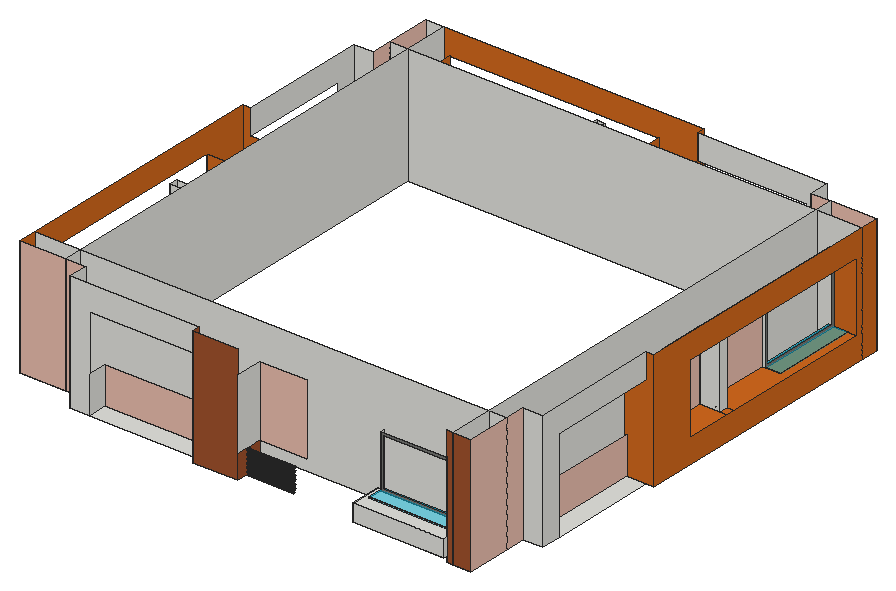
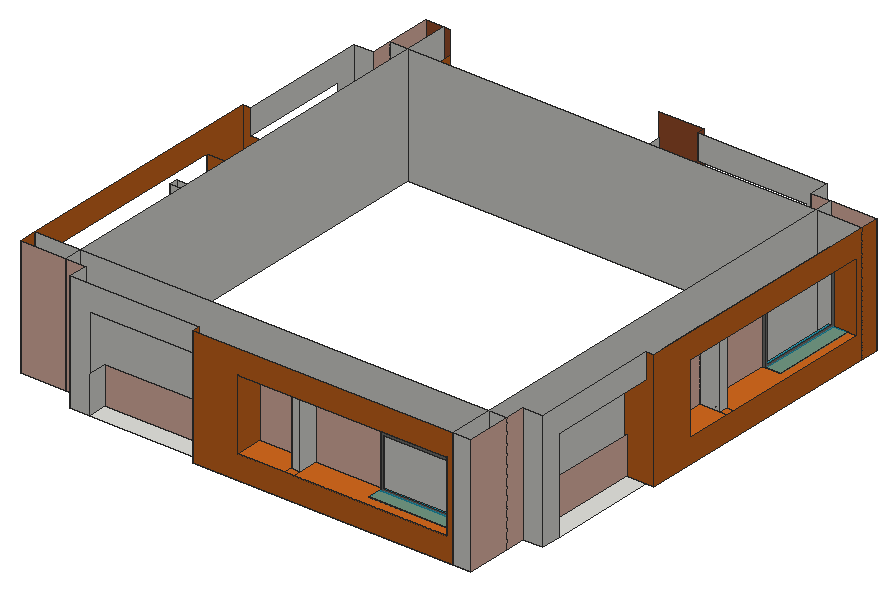
# SketchUp Ruby script. Lengths in inches.
U = 1.inch
M = Sketchup.active_model
def pt(a) = Geom::Point3d.new(a.map { |v| v * U })
def face(e, loops, mat)
  f = e.add_face(loops[0].map { |a| pt(a) })
  loops[1..].each { |l| e.add_face(l.map { |a| pt(a) }).erase! }
  f.material = f.back_material = mat if mat
  f
end
# faces: each face lists its corners as indices into pts; further lists are holes
def faces(e, pts, list, mat = nil) = list.each { |f| face(e, (f[0].is_a?(Array) ? f : [f]).map { |l| l.map { |i| pts[i] } }, mat) }
# xy, xz, yz: faces in a plane at the given z, y or x. An outline is a flat list of corners, or four numbers for a rectangle; further outlines are holes
def ring(l) = l.size == 4 ? [[l[0], l[1]], [l[2], l[1]], [l[2], l[3]], [l[0], l[3]]] : l.each_slice(2).to_a
def flat(e, list, mat, &to3) = list.each { |f| face(e, (f[0].is_a?(Array) ? f : [f]).map { |l| ring(l).map { |u, v| to3.(u, v) } }, mat) }
def xy(e, z, list, mat = nil) = flat(e, list, mat) { |x, y| [x, y, z] }
def xz(e, y, list, mat = nil) = flat(e, list, mat) { |x, z| [x, y, z] }
def yz(e, x, list, mat = nil) = flat(e, list, mat) { |y, z| [x, y, z] }
def lines(e, pts, list) = list.each { |a, b| e.add_line(pt(pts[a]), pt(pts[b])) }
# prism: a flat outline (further loops are holes) pulled along v
def prism(e, loops, v, mat = nil)
  f = face(e, loops, mat); d = Geom::Vector3d.new(v.map { |x| x * U })
  f.pushpull(f.normal.samedirection?(d) ? d.length : -d.length)
end
def box(e, o, s, mat = nil) = prism(e, [[o, [o[0] + s[0], o[1], o[2]], [o[0] + s[0], o[1] + s[1], o[2]], [o[0], o[1] + s[1], o[2]]]], [0, 0, s[2]], mat)
def at(x, y, z, deg = 0) = Geom::Transformation.translation(pt([x, y, z])) * Geom::Transformation.rotation(ORIGIN, Z_AXIS, deg.degrees)
def axes(o, x, y, z) = Geom::Transformation.new([*x, 0, *y, 0, *z, 0, *pt(o).to_a, 1])
def part(name) = M.definitions.add(name)
# library, detail: a bought-in or finely detailed component or shape, given as its bounding box
def library(name, o, s) = part(name).tap { |d| box(d.entities, o, s) }
def detail(e, o, s) = box(e.add_group.entities, o, s)
def put(e, d, t, mat = nil) = e.add_instance(d, t).tap { |i| i.material = mat if mat }
def group(e, t, mat = nil) = e.add_group.tap { |g| g.transformation = t; g.material = mat if mat }.entities
root = M.entities
M.materials.add("[0041_Chocolate]").color = [210, 105, 30]
M.materials.add("[0042_Sienna]").color = [160, 82, 45]
M.materials.add("[0119_RosyBrown]").color = [234, 190, 174]
M.materials.add("[Metal Seamed]").color = [118, 119, 115]
M.materials.add("[Translucent Glass Tinted]").color = [8, 201, 241]
M.materials["[Translucent Glass Tinted]"].alpha = 0.48
c1 = part("Altan")
box(c1.entities,[0,0,0],[118.11,59.06,3.9375])
prism(root,[[[1139,96.8125,797.98],[1414.89,97.68,797.98],[1415.2,0.87,797.98],[1139.3,0,797.98]]],[0,0,52.19])
xy(root,780,[[1434.3125,12.8125,1488,150.5],[306.65,36.8125,641.22,96.8125],[48,96.8125,185.6875,150.5],[48,150.5,185.6875,150.5,185.6875,1399.125,132,1399.125,132,1338.16,72,1338.16,72,1278.16,132,1278.16,132,943.59,48,943.59],[1434.3125,150.5,1488,150.5,1488,211.46,1548,211.46,1548,271.47,1488,271.47,1488,606.03,1572,606.03,1572,1399.125,1434.3125,1399.125],
  [1488,271.47,1548,606.03],[72,943.59,132,1278.16],[132,1399.125,185.6875,1536.8125],[185.6875,1399.125,1434.3125,1399.125,1434.3125,1452.8125,1373.35,1452.8125,1373.35,1512.8125,1313.35,1512.8125,1313.35,1452.8125,978.78,1452.8125,978.78,1536.8125,185.6875,1536.8125],[1434.3125,1399.125,1572,1452.8125],
  [978.78,1452.8125,1313.35,1512.8125]])
xy(root,853.11,[[72,636.29,132,662.8],[1488,886.83,1548,913.33],[671.48,1452.8125,697.99,1512.8125]])
xy(root,853.11,[[48,169.92,120,169.92,120,429.61,132,429.61,132,636.29,48,636.29],[48,636.29,72,662.8],[48,662.8,132,806.17],[1488,743.45,1572,886.83],[1548,886.83,1572,913.33],
  [1488,913.33,1572,913.33,1572,1379.7,1500,1379.7,1500,1120.01,1488,1120.01],[464.8,1452.8125,671.48,1452.8125,671.48,1536.8125,205.11,1536.8125,205.11,1464.8125,464.8,1464.8125],[697.99,1452.8125,841.36,1536.8125],[671.48,1512.8125,697.99,1536.8125]],"[0041_Chocolate]")
xy(root,853.11,[[1155.2,84.8125,1414.89,96.8125]],"[0042_Sienna]")
xz(root,12.8125,[[641.22,780,778.64,1140],[1414.89,780,1434.3125,1140],[1434.3125,780,1488,1140]],"[0042_Sienna]")
xz(root,36.8125,[[246.65,780,306.65,780,306.65,1062.625,641.22,1062.625,641.22,1140,246.65,1140]])
xz(root,84.8125,[[[1155.2,853.11,1414.89,1013.61],[1161.2,859.11,1408.89,1007.61]]],"[Metal Seamed]")
xz(root,96.8125,[[48,780,185.6875,1140],[185.6875,780,246.65,1140],[306.65,780,641.22,893.76],[778.64,853.11,922.01,1066.89]],"[0119_RosyBrown]")
xz(root,150.5,[[48,780,1488,1140]])
xz(root,169.92,[[48,853.11,48,1066.89,132,1066.89,132,1013.61,120,1013.61,120,853.11]],"[0041_Chocolate]")
xz(root,211.46,[[1488,780,1548,1140]])
xz(root,271.47,[[1488,780,1548,893.76]])
xz(root,429.61,[[120,853.11,132,1013.61]],"[Metal Seamed]")
xz(root,606.03,[[1488,780,1572,780,1572,1140,1548,1140,1548,1062.625,1482,1062.625,1482,893.76,1488,893.76]],"[0041_Chocolate]")
xz(root,636.29,[[72,853.11,132,1066.89]])
xz(root,662.8,[[[72,853.11,132,1066.89],[83.53,858.02,84.48,858.14,85.37,858.51,86.13,859.1,86.72,859.86,87.09,860.75,87.21,861.7,87.09,862.66,86.72,863.55,86.13,864.3125,85.37,864.9,84.48,865.27,83.53,865.39,82.57,865.27,81.68,864.9,80.92,864.3125,80.33,863.55,79.97,862.66,79.84,861.7,79.97,860.75,80.33,859.86,80.92,859.1,81.68,858.51,82.57,858.14]]])
xz(root,743.45,[[[1488,853.11,1572,1066.89],[1536.47,858.02,1537.43,858.14,1538.32,858.51,1539.08,859.1,1539.67,859.86,1540.03,860.75,1540.16,861.7,1540.03,862.66,1539.67,863.55,1539.08,864.3125,1538.32,864.9,1537.43,865.27,1536.47,865.39,1535.52,865.27,1534.63,864.9,1533.87,864.3125,1533.28,863.55,1532.91,862.66,1532.79,861.7,1532.91,860.75,1533.28,859.86,1533.87,859.1,1534.63,858.51,1535.52,858.14]]],"[0041_Chocolate]")
xz(root,806.17,[[[48,853.11,132,1066.89],[83.53,858.02,82.57,858.14,81.68,858.51,80.92,859.1,80.33,859.86,79.97,860.75,79.84,861.7,79.97,862.66,80.33,863.55,80.92,864.3125,81.68,864.9,82.57,865.27,83.53,865.39,84.48,865.27,85.37,864.9,86.13,864.3125,86.72,863.55,87.09,862.66,87.21,861.7,87.09,860.75,86.72,859.86,86.13,859.1,85.37,858.51,84.48,858.14]]],"[0041_Chocolate]")
xz(root,886.83,[[[1488,853.11,1548,1066.89],[1536.47,858.02,1535.52,858.14,1534.63,858.51,1533.87,859.1,1533.28,859.86,1532.91,860.75,1532.79,861.7,1532.91,862.66,1533.28,863.55,1533.87,864.3125,1534.63,864.9,1535.52,865.27,1536.47,865.39,1537.43,865.27,1538.32,864.9,1539.08,864.3125,1539.67,863.55,1540.03,862.66,1540.16,861.7,1540.03,860.75,1539.67,859.86,1539.08,859.1,1538.32,858.51,1537.43,858.14]]])
xz(root,913.33,[[1488,853.11,1548,1066.89]])
xz(root,943.59,[[48,780,48,1140,72,1140,72,1062.625,138,1062.625,138,893.76,132,893.76,132,780]],"[0041_Chocolate]")
xz(root,1120.01,[[1488,853.11,1500,1013.61]])
xz(root,1278.16,[[72,780,132,893.76]])
xz(root,1338.16,[[72,780,132,1140]])
xz(root,1379.7,[[1500,853.11,1572,853.11,1572,1066.89,1488,1066.89,1488,1013.61,1500,1013.61]],"[0041_Chocolate]")
xz(root,1399.125,[[132,780,1572,1140]])
xz(root,1452.8125,[[671.48,853.11,697.99,1066.89]])
xz(root,1452.8125,[[978.78,780,1313.35,893.76],[1373.35,780,1434.3125,1140],[1434.3125,780,1572,1140],[464.8,853.11,464.8,1013.61,205.11,1013.61,205.11,1066.89,671.48,1066.89,671.48,853.11],[697.99,853.11,841.36,1066.89]],"[0119_RosyBrown]")
xz(root,1464.8125,[[[205.11,853.11,464.8,1013.61],[211.11,859.11,458.8,1007.61]]],"[Metal Seamed]")
xz(root,1512.8125,[[1313.35,780,1313.35,1062.625,978.78,1062.625,978.78,1140,1373.35,1140,1373.35,780],[671.48,853.11,697.99,1066.89]])
xz(root,1536.8125,[[132,780,185.6875,1140]])
xz(root,1536.8125,[[[185.6875,780,978.78,1140],[205.11,853.11,841.36,1066.89]]],"[0041_Chocolate]")
yz(root,48,[[96.8125,780,150.5,1140],[[150.5,780,943.59,1140],[169.92,853.11,806.17,1066.89]]],"[0041_Chocolate]")
yz(root,72,[[1278.16,780,1278.16,1062.625,943.59,1062.625,943.59,1140,1338.16,1140,1338.16,780],[636.29,853.11,662.8,1066.89]])
yz(root,120,[[[169.92,853.11,429.61,1013.61],[175.92,859.11,423.61,1007.61]]],"[Metal Seamed]")
yz(root,132,[[636.29,853.11,662.8,1066.89]])
yz(root,132,[[943.59,780,1278.16,893.76],[1338.16,780,1399.125,1140],[1399.125,780,1536.8125,1140],[429.61,853.11,429.61,1013.61,169.92,1013.61,169.92,1066.89,636.29,1066.89,636.29,853.11],[662.8,853.11,806.17,1066.89]],"[0119_RosyBrown]")
yz(root,185.6875,[[96.8125,780,1536.8125,1140]])
yz(root,205.11,[[1464.8125,853.11,1536.8125,853.11,1536.8125,1066.89,1452.8125,1066.89,1452.8125,1013.61,1464.8125,1013.61]],"[0041_Chocolate]")
yz(root,246.65,[[36.8125,780,96.8125,1140]])
yz(root,306.65,[[36.8125,780,96.8125,893.76]])
yz(root,464.8,[[1452.8125,853.11,1464.8125,1013.61]])
yz(root,641.22,[[12.8125,780,12.8125,1140,36.8125,1140,36.8125,1062.625,102.8125,1062.625,102.8125,893.76,96.8125,893.76,96.8125,780]],"[0042_Sienna]")
yz(root,671.48,[[1452.8125,853.11,1512.8125,1066.89]])
yz(root,697.99,[[[1452.8125,853.11,1512.8125,1066.89],[1501.28,858.02,1500.33,858.14,1499.44,858.51,1498.68,859.1,1498.09,859.86,1497.72,860.75,1497.6,861.7,1497.72,862.66,1498.09,863.55,1498.68,864.3125,1499.44,864.9,1500.33,865.27,1501.28,865.39,1502.24,865.27,1503.13,864.9,1503.89,864.3125,1504.48,863.55,1504.85,862.66,1504.97,861.7,1504.85,860.75,1504.48,859.86,1503.89,859.1,1503.13,858.51,1502.24,858.14]]])
yz(root,778.64,[[[12.8125,853.11,47.01,853.11,47.38,853.27,48.34,853.39,49.29,853.27,49.67,853.11,96.8125,853.11,96.8125,1066.89,51.8,1066.89,51.9,1066.66,52.03,1065.7,51.9,1064.75,51.53,1063.86,50.95,1063.1,50.18,1062.51,49.29,1062.14,48.34,1062.02,47.38,1062.14,46.5,1062.51,45.73,1063.1,45.15,1063.86,44.78,1064.75,44.65,1065.7,44.78,1066.66,44.875,1066.89,12.8125,1066.89],[48.34,858.02,47.38,858.14,46.5,858.51,45.73,859.1,45.15,859.86,44.78,860.75,44.65,861.7,44.78,862.66,45.15,863.55,45.73,864.3125,46.5,864.9,47.38,865.27,48.34,865.39,49.29,865.27,50.18,864.9,50.95,864.3125,51.53,863.55,51.9,862.66,52.03,861.7,51.9,860.75,51.53,859.86,50.95,859.1,50.18,858.51,49.29,858.14]],[47.01,853.11,49.67,853.11,49.29,853.27,48.34,853.39,47.38,853.27]])
yz(root,778.64,[[12.8125,780,45.49,780,45.73,780.3125,46.5,780.9,47.38,781.27,48.34,781.39,49.29,781.27,50.18,780.9,50.95,780.3125,51.19,780,96.8125,780,96.8125,853.11,49.67,853.11,50.18,852.9,50.95,852.3125,51.53,851.55,51.9,850.66,52.03,849.7,51.9,848.75,51.53,847.86,50.95,847.1,50.18,846.51,49.29,846.14,48.34,846.02,47.38,846.14,46.5,846.51,45.73,847.1,45.15,847.86,44.78,848.75,44.65,849.7,44.78,850.66,45.15,851.55,45.73,852.3125,46.5,852.9,47.01,853.11,12.8125,853.11],[45.49,780,51.19,780,50.95,780.3125,50.18,780.9,49.29,781.27,48.34,781.39,47.38,781.27,46.5,780.9,45.73,780.3125],[48.34,846.02,49.29,846.14,50.18,846.51,50.95,847.1,51.53,847.86,51.9,848.75,52.03,849.7,51.9,850.66,51.53,851.55,50.95,852.3125,50.18,852.9,49.67,853.11,47.01,853.11,46.5,852.9,45.73,852.3125,45.15,851.55,44.78,850.66,44.65,849.7,44.78,848.75,45.15,847.86,45.73,847.1,46.5,846.51,47.38,846.14]],"[0042_Sienna]")
yz(root,841.36,[[[1452.8125,853.11,1536.8125,1066.89],[1501.28,858.02,1502.24,858.14,1503.13,858.51,1503.89,859.1,1504.48,859.86,1504.85,860.75,1504.97,861.7,1504.85,862.66,1504.48,863.55,1503.89,864.3125,1503.13,864.9,1502.24,865.27,1501.28,865.39,1500.33,865.27,1499.44,864.9,1498.68,864.3125,1498.09,863.55,1497.72,862.66,1497.6,861.7,1497.72,860.75,1498.09,859.86,1498.68,859.1,1499.44,858.51,1500.33,858.14]]],"[0041_Chocolate]")
yz(root,978.78,[[1452.8125,780,1536.8125,780,1536.8125,1140,1512.8125,1140,1512.8125,1062.625,1446.8125,1062.625,1446.8125,893.76,1452.8125,893.76]],"[0041_Chocolate]")
yz(root,1155.2,[[84.8125,853.11,96.8125,1013.61]])
yz(root,1313.35,[[1452.8125,780,1512.8125,893.76]])
yz(root,1373.35,[[1452.8125,780,1512.8125,1140]])
yz(root,1414.89,[[12.8125,853.11,12.8125,1066.89,96.8125,1066.89,96.8125,1013.61,84.8125,1013.61,84.8125,853.11]],"[0041_Chocolate]")
yz(root,1414.89,[[12.8125,780,96.8125,853.11]],"[0042_Sienna]")
yz(root,1434.3125,[[12.8125,780,1452.8125,1140]])
yz(root,1488,[[886.83,853.11,913.33,1066.89]])
yz(root,1488,[[12.8125,780,150.5,1140],[150.5,780,211.46,1140],[271.47,780,606.03,893.76],[743.45,853.11,886.83,1066.89],[913.33,853.11,1120.01,853.11,1120.01,1013.61,1379.7,1013.61,1379.7,1066.89,913.33,1066.89]],"[0119_RosyBrown]")
yz(root,1500,[[[1120.01,853.11,1379.7,1013.61],[1126.01,859.11,1373.7,1007.61]]],"[Metal Seamed]")
yz(root,1548,[[211.46,780,271.47,780,271.47,1062.625,606.03,1062.625,606.03,1140,211.46,1140],[886.83,853.11,913.33,1066.89]])
yz(root,1572,[[[606.03,780,1399.125,1140],[743.45,853.11,1379.7,1066.89]],[1399.125,780,1452.8125,1140]],"[0041_Chocolate]")
p = [[922.01,45.15,779.55],[922.01,45.73,780.3125],[778.64,45.73,780.3125],[778.64,45.49,780],[778.64,45.15,779.55],[922.01,50.95,780.3125],
  [922.01,51.53,779.55],[778.64,51.53,779.55],[778.64,51.19,780],[778.64,50.95,780.3125],[922.01,46.5,780.9],[778.64,46.5,780.9],
  [922.01,50.18,780.9],[778.64,50.18,780.9],[922.01,47.38,781.27],[778.64,47.38,781.27],[922.01,49.29,781.27],[778.64,49.29,781.27],
  [922.01,48.34,781.39],[778.64,48.34,781.39],[922.01,48.34,786.02],[922.01,47.38,786.14],[778.64,47.38,786.14],[778.64,48.34,786.02],
  [922.01,49.29,786.14],[778.64,49.29,786.14],[922.01,46.5,786.51],[778.64,46.5,786.51],[922.01,50.18,786.51],[778.64,50.18,786.51],
  [922.01,45.73,787.1],[778.64,45.73,787.1],[922.01,50.95,787.1],[778.64,50.95,787.1],[922.01,45.15,787.86],[778.64,45.15,787.86],
  [922.01,51.53,787.86],[778.64,51.53,787.86],[922.01,44.78,788.75],[778.64,44.78,788.75],[922.01,51.9,788.75],[778.64,51.9,788.75],
  [922.01,44.65,789.7],[778.64,44.65,789.7],[922.01,52.03,789.7],[778.64,52.03,789.7],[922.01,44.78,790.66],[778.64,44.78,790.66],
  [922.01,51.9,790.66],[778.64,51.9,790.66],[922.01,45.15,791.55],[778.64,45.15,791.55],[922.01,51.53,791.55],[778.64,51.53,791.55],
  [922.01,45.73,792.3125],[778.64,45.73,792.3125],[922.01,50.95,792.3125],[778.64,50.95,792.3125],[922.01,46.5,792.9],[778.64,46.5,792.9],
  [922.01,50.18,792.9],[778.64,50.18,792.9],[922.01,47.38,793.27],[778.64,47.38,793.27],[922.01,49.29,793.27],[778.64,49.29,793.27],
  [922.01,48.34,793.39],[778.64,48.34,793.39],[922.01,48.34,798.02],[922.01,47.38,798.14],[778.64,47.38,798.14],[778.64,48.34,798.02],
  [922.01,49.29,798.14],[778.64,49.29,798.14],[922.01,46.5,798.51],[778.64,46.5,798.51],[922.01,50.18,798.51],[778.64,50.18,798.51],
  [922.01,45.73,799.1],[778.64,45.73,799.1],[922.01,50.95,799.1],[778.64,50.95,799.1],[922.01,45.15,799.86],[778.64,45.15,799.86],
  [922.01,51.53,799.86],[778.64,51.53,799.86],[922.01,44.78,800.75],[778.64,44.78,800.75],[922.01,51.9,800.75],[778.64,51.9,800.75],
  [922.01,44.65,801.7],[778.64,44.65,801.7],[922.01,52.03,801.7],[778.64,52.03,801.7],[922.01,44.78,802.66],[778.64,44.78,802.66],
  [922.01,51.9,802.66],[778.64,51.9,802.66],[922.01,45.15,803.55],[778.64,45.15,803.55],[922.01,51.53,803.55],[778.64,51.53,803.55],
  [922.01,45.73,804.3125],[778.64,45.73,804.3125],[922.01,50.95,804.3125],[778.64,50.95,804.3125],[922.01,46.5,804.9],[778.64,46.5,804.9],
  [922.01,50.18,804.9],[778.64,50.18,804.9],[922.01,47.38,805.27],[778.64,47.38,805.27],[922.01,49.29,805.27],[778.64,49.29,805.27],
  [922.01,48.34,805.39],[778.64,48.34,805.39],[922.01,48.34,810.02],[922.01,47.38,810.14],[778.64,47.38,810.14],[778.64,48.34,810.02],
  [922.01,49.29,810.14],[778.64,49.29,810.14],[922.01,46.5,810.51],[778.64,46.5,810.51],[922.01,50.18,810.51],[778.64,50.18,810.51],
  [922.01,45.73,811.1],[778.64,45.73,811.1],[922.01,50.95,811.1],[778.64,50.95,811.1],[922.01,45.15,811.86],[778.64,45.15,811.86],
  [922.01,51.53,811.86],[778.64,51.53,811.86],[922.01,44.78,812.75],[778.64,44.78,812.75],[922.01,51.9,812.75],[778.64,51.9,812.75],
  [922.01,44.65,813.7],[778.64,44.65,813.7],[922.01,52.03,813.7],[778.64,52.03,813.7],[922.01,44.78,814.66],[778.64,44.78,814.66],
  [922.01,51.9,814.66],[778.64,51.9,814.66],[922.01,45.15,815.55],[778.64,45.15,815.55],[922.01,51.53,815.55],[778.64,51.53,815.55],
  [922.01,45.73,816.3125],[778.64,45.73,816.3125],[922.01,50.95,816.3125],[778.64,50.95,816.3125],[922.01,46.5,816.9],[778.64,46.5,816.9],
  [922.01,50.18,816.9],[778.64,50.18,816.9],[922.01,47.38,817.27],[778.64,47.38,817.27],[922.01,49.29,817.27],[778.64,49.29,817.27],
  [922.01,48.34,817.39],[778.64,48.34,817.39],[922.01,48.34,822.02],[922.01,47.38,822.14],[778.64,47.38,822.14],[778.64,48.34,822.02],
  [922.01,49.29,822.14],[778.64,49.29,822.14],[922.01,46.5,822.51],[778.64,46.5,822.51],[922.01,50.18,822.51],[778.64,50.18,822.51],
  [922.01,45.73,823.1],[778.64,45.73,823.1],[922.01,50.95,823.1],[778.64,50.95,823.1],[922.01,45.15,823.86],[778.64,45.15,823.86],
  [922.01,51.53,823.86],[778.64,51.53,823.86],[922.01,44.78,824.75],[778.64,44.78,824.75],[922.01,51.9,824.75],[778.64,51.9,824.75],
  [922.01,44.65,825.7],[778.64,44.65,825.7],[922.01,52.03,825.7],[778.64,52.03,825.7],[922.01,44.78,826.66],[778.64,44.78,826.66],
  [922.01,51.9,826.66],[778.64,51.9,826.66],[922.01,45.15,827.55],[778.64,45.15,827.55],[922.01,51.53,827.55],[778.64,51.53,827.55],
  [922.01,45.73,828.3125],[778.64,45.73,828.3125],[922.01,50.95,828.3125],[778.64,50.95,828.3125],[922.01,46.5,828.9],[778.64,46.5,828.9],
  [922.01,50.18,828.9],[778.64,50.18,828.9],[922.01,47.38,829.27],[778.64,47.38,829.27],[922.01,49.29,829.27],[778.64,49.29,829.27],
  [922.01,48.34,829.39],[778.64,48.34,829.39],[922.01,48.34,834.02],[922.01,47.38,834.14],[778.64,47.38,834.14],[778.64,48.34,834.02],
  [922.01,49.29,834.14],[778.64,49.29,834.14],[922.01,46.5,834.51],[778.64,46.5,834.51],[922.01,50.18,834.51],[778.64,50.18,834.51],
  [922.01,45.73,835.1],[778.64,45.73,835.1],[922.01,50.95,835.1],[778.64,50.95,835.1],[922.01,45.15,835.86],[778.64,45.15,835.86],
  [922.01,51.53,835.86],[778.64,51.53,835.86],[922.01,44.78,836.75],[778.64,44.78,836.75],[922.01,51.9,836.75],[778.64,51.9,836.75],
  [922.01,44.65,837.7],[778.64,44.65,837.7],[922.01,52.03,837.7],[778.64,52.03,837.7],[922.01,44.78,838.66],[778.64,44.78,838.66],
  [922.01,51.9,838.66],[778.64,51.9,838.66],[922.01,45.15,839.55],[778.64,45.15,839.55],[922.01,51.53,839.55],[778.64,51.53,839.55],
  [922.01,45.73,840.3125],[778.64,45.73,840.3125],[922.01,50.95,840.3125],[778.64,50.95,840.3125],[922.01,46.5,840.9],[778.64,46.5,840.9],
  [922.01,50.18,840.9],[778.64,50.18,840.9],[922.01,47.38,841.27],[778.64,47.38,841.27],[922.01,49.29,841.27],[778.64,49.29,841.27],
  [922.01,48.34,841.39],[778.64,48.34,841.39],[922.01,48.34,846.02],[922.01,47.38,846.14],[778.64,47.38,846.14],[778.64,48.34,846.02],
  [922.01,49.29,846.14],[778.64,49.29,846.14],[922.01,46.5,846.51],[778.64,46.5,846.51],[922.01,50.18,846.51],[778.64,50.18,846.51],
  [922.01,45.73,847.1],[778.64,45.73,847.1],[922.01,50.95,847.1],[778.64,50.95,847.1],[922.01,45.15,847.86],[778.64,45.15,847.86],
  [922.01,51.53,847.86],[778.64,51.53,847.86],[922.01,44.78,848.75],[778.64,44.78,848.75],[922.01,51.9,848.75],[778.64,51.9,848.75],
  [922.01,44.65,849.7],[778.64,44.65,849.7],[922.01,52.03,849.7],[778.64,52.03,849.7],[922.01,44.78,850.66],[778.64,44.78,850.66],
  [922.01,51.9,850.66],[778.64,51.9,850.66],[922.01,45.15,851.55],[778.64,45.15,851.55],[922.01,51.53,851.55],[778.64,51.53,851.55],
  [922.01,45.73,852.3125],[778.64,45.73,852.3125],[922.01,50.95,852.3125],[778.64,50.95,852.3125],[922.01,46.5,852.9],[778.64,46.5,852.9],
  [922.01,50.18,852.9],[778.64,50.18,852.9],[922.01,47.38,853.27],[778.64,47.38,853.27],[778.64,47.01,853.11],[922.01,49.29,853.27],
  [778.64,49.67,853.11],[778.64,49.29,853.27],[922.01,48.34,853.39],[778.64,48.34,853.39]]
faces(root,p,[[0,1,2,3,4],[5,6,7,8,9],[1,10,11,2],[12,5,9,13],[10,14,15,11],[16,12,13,17],[14,18,19,15],[18,16,17,19],
  [20,21,22,23],[24,20,23,25],[21,26,27,22],[28,24,25,29],[26,30,31,27],[32,28,29,33],[30,34,35,31],[36,32,33,37],
  [34,38,39,35],[40,36,37,41],[38,42,43,39],[44,40,41,45],[42,46,47,43],[48,44,45,49],[46,50,51,47],[52,48,49,53],
  [50,54,55,51],[56,52,53,57],[54,58,59,55],[60,56,57,61],[58,62,63,59],[64,60,61,65],[62,66,67,63],[66,64,65,67],
  [68,69,70,71],[72,68,71,73],[69,74,75,70],[76,72,73,77],[74,78,79,75],[80,76,77,81],[78,82,83,79],[84,80,81,85],
  [82,86,87,83],[88,84,85,89],[86,90,91,87],[92,88,89,93],[90,94,95,91],[96,92,93,97],[94,98,99,95],[100,96,97,101],
  [98,102,103,99],[104,100,101,105],[102,106,107,103],[108,104,105,109],[106,110,111,107],[112,108,109,113],[110,114,115,111],[114,112,113,115],
  [116,117,118,119],[120,116,119,121],[117,122,123,118],[124,120,121,125],[122,126,127,123],[128,124,125,129],[126,130,131,127],[132,128,129,133],
  [130,134,135,131],[136,132,133,137],[134,138,139,135],[140,136,137,141],[138,142,143,139],[144,140,141,145],[142,146,147,143],[148,144,145,149],
  [146,150,151,147],[152,148,149,153],[150,154,155,151],[156,152,153,157],[154,158,159,155],[160,156,157,161],[158,162,163,159],[162,160,161,163],
  [164,165,166,167],[168,164,167,169],[165,170,171,166],[172,168,169,173],[170,174,175,171],[176,172,173,177],[174,178,179,175],[180,176,177,181],
  [178,182,183,179],[184,180,181,185],[182,186,187,183],[188,184,185,189],[186,190,191,187],[192,188,189,193],[190,194,195,191],[196,192,193,197],
  [194,198,199,195],[200,196,197,201],[198,202,203,199],[204,200,201,205],[202,206,207,203],[208,204,205,209],[206,210,211,207],[210,208,209,211],
  [212,213,214,215],[216,212,215,217],[213,218,219,214],[220,216,217,221],[218,222,223,219],[224,220,221,225],[222,226,227,223],[228,224,225,229],
  [226,230,231,227],[232,228,229,233],[230,234,235,231],[236,232,233,237],[234,238,239,235],[240,236,237,241],[238,242,243,239],[244,240,241,245],
  [242,246,247,243],[248,244,245,249],[246,250,251,247],[252,248,249,253],[250,254,255,251],[256,252,253,257],[254,258,259,255],[258,256,257,259],
  [260,261,262,263],[264,260,263,265],[261,266,267,262],[268,264,265,269],[266,270,271,267],[272,268,269,273],[270,274,275,271],[276,272,273,277],
  [274,278,279,275],[280,276,277,281],[278,282,283,279],[284,280,281,285],[282,286,287,283],[288,284,285,289],[286,290,291,287],[292,288,289,293],
  [290,294,295,291],[296,292,293,297],[294,298,299,295],[300,296,297,301],[298,302,303,304,299],[305,300,301,306,307],[302,308,309,303],[308,305,307,309]])
put(root,c1,axes([1487.13,1379.7,849.17],[0,-2.19843,0],[1,0,0],[0,0,1.5]),"[Translucent Glass Tinted]")
put(root,c1,axes([132.87,169.92,849.17],[0,2.19843,0],[-1,0,0],[0,0,1.5]),"[Translucent Glass Tinted]")
put(root,c1,axes([205.11,1451.94,849.17],[2.19843,0,0],[0,1,0],[0,0,1.5]),"[Translucent Glass Tinted]")
put(root,c1,axes([1414.89,97.68,849.17],[-2.19843,0,0],[0,-1,0],[0,0,1.5]),"[Translucent Glass Tinted]")
